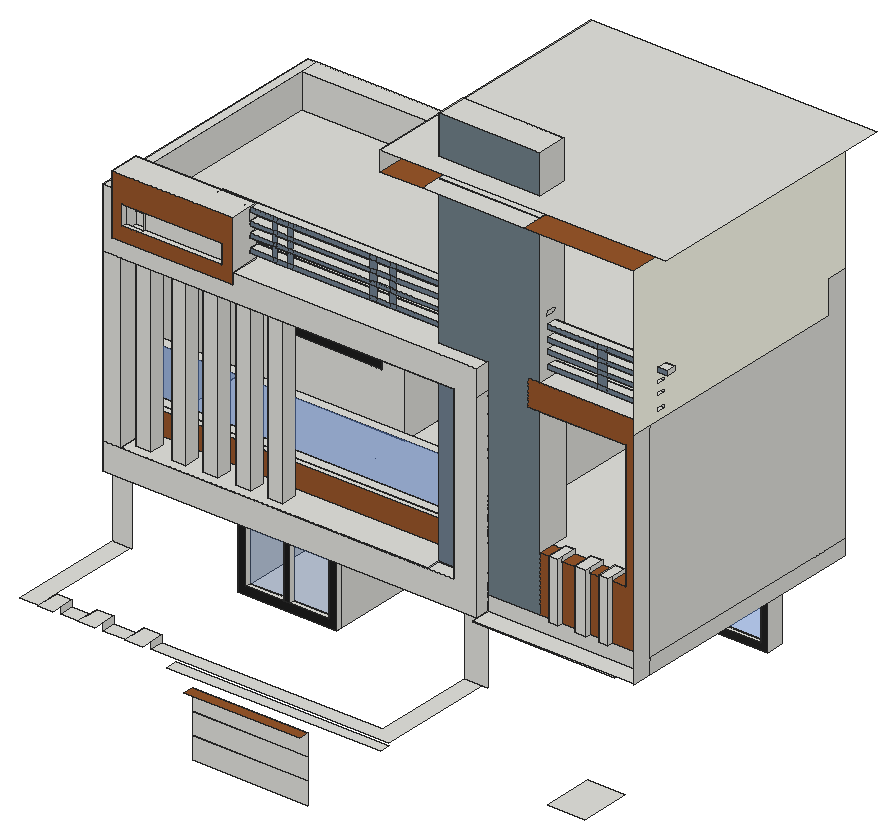
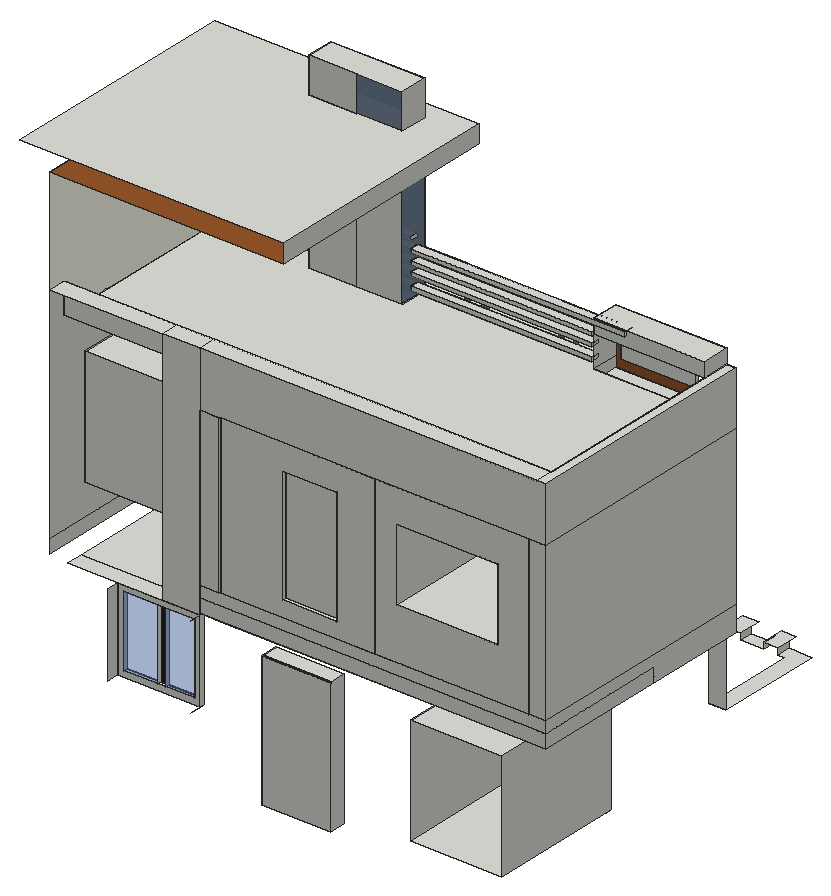
# SketchUp Ruby script. Lengths in inches.
U = 1.inch
M = Sketchup.active_model
def pt(a) = Geom::Point3d.new(a.map { |v| v * U })
def face(e, loops, mat)
  f = e.add_face(loops[0].map { |a| pt(a) })
  loops[1..].each { |l| e.add_face(l.map { |a| pt(a) }).erase! }
  f.material = f.back_material = mat if mat
  f
end
# faces: each face lists its corners as indices into pts; further lists are holes
def faces(e, pts, list, mat = nil) = list.each { |f| face(e, (f[0].is_a?(Array) ? f : [f]).map { |l| l.map { |i| pts[i] } }, mat) }
# xy, xz, yz: faces in a plane at the given z, y or x. An outline is a flat list of corners, or four numbers for a rectangle; further outlines are holes
def ring(l) = l.size == 4 ? [[l[0], l[1]], [l[2], l[1]], [l[2], l[3]], [l[0], l[3]]] : l.each_slice(2).to_a
def flat(e, list, mat, &to3) = list.each { |f| face(e, (f[0].is_a?(Array) ? f : [f]).map { |l| ring(l).map { |u, v| to3.(u, v) } }, mat) }
def xy(e, z, list, mat = nil) = flat(e, list, mat) { |x, y| [x, y, z] }
def xz(e, y, list, mat = nil) = flat(e, list, mat) { |x, z| [x, y, z] }
def yz(e, x, list, mat = nil) = flat(e, list, mat) { |y, z| [x, y, z] }
def lines(e, pts, list) = list.each { |a, b| e.add_line(pt(pts[a]), pt(pts[b])) }
# prism: a flat outline (further loops are holes) pulled along v
def prism(e, loops, v, mat = nil)
  f = face(e, loops, mat); d = Geom::Vector3d.new(v.map { |x| x * U })
  f.pushpull(f.normal.samedirection?(d) ? d.length : -d.length)
end
def box(e, o, s, mat = nil) = prism(e, [[o, [o[0] + s[0], o[1], o[2]], [o[0] + s[0], o[1] + s[1], o[2]], [o[0], o[1] + s[1], o[2]]]], [0, 0, s[2]], mat)
def at(x, y, z, deg = 0) = Geom::Transformation.translation(pt([x, y, z])) * Geom::Transformation.rotation(ORIGIN, Z_AXIS, deg.degrees)
def axes(o, x, y, z) = Geom::Transformation.new([*x, 0, *y, 0, *z, 0, *pt(o).to_a, 1])
def part(name) = M.definitions.add(name)
# library, detail: a bought-in or finely detailed component or shape, given as its bounding box
def library(name, o, s) = part(name).tap { |d| box(d.entities, o, s) }
def detail(e, o, s) = box(e.add_group.entities, o, s)
def put(e, d, t, mat = nil) = e.add_instance(d, t).tap { |i| i.material = mat if mat }
def group(e, t, mat = nil) = e.add_group.tap { |g| g.transformation = t; g.material = mat if mat }.entities
root = M.entities
M.materials.add("[0053_Ivory]").color = [255, 255, 240]
M.materials.add("[0111_SlateGray]").color = [112, 130, 152]
M.materials["[0111_SlateGray]"].alpha = 0.95
M.materials.add("[0111_SlateGray]1").color = [112, 128, 136]
M.materials.add("[0111_SlateGray]2").color = [112, 128, 144]
M.materials.add("[0136_Charcoal]").color = [35, 35, 35]
M.materials.add("[Color M08]").color = [30, 30, 30]
M.materials.add("[Translucent Glass Blue]").color = [100, 149, 237]
M.materials["[Translucent Glass Blue]"].alpha = 0.25
M.materials.add("[Translucent Glass Blue]1").color = [100, 149, 237]
M.materials["[Translucent Glass Blue]1"].alpha = 0.27
M.materials.add("[Translucent Glass Blue]2").color = [100, 149, 237]
M.materials["[Translucent Glass Blue]2"].alpha = 0.48
M.materials.add("[Translucent_Glass_Blue]1").color = [100, 149, 237]
M.materials["[Translucent_Glass_Blue]1"].alpha = 0.5
M.materials.add("[Wood Cherry Original]").color = [152, 86, 42]
c1 = part("DOOR12")
g1 = group(c1.entities,at(114.73,28.14,-0.51))
g2 = group(g1,at(0,0,0))
box(g2,[0,0,0],[36,0.5,77.7])
xy(root,4.04,[[120.48,208.05,157.11,217.05]])
xy(root,14.85,[[29.05,144.8,77.86,217.05]])
xy(root,40.28,[[90.86,34.4375,147.74,39.75]],"[Wood Cherry Original]")
xy(root,48.65,[[82.49,34.4375,187.77,39.75]])
xy(root,49.9375,[[5.71,39.75,18.06,39.75,18.06,46.62,14.21,46.62,14.21,97.05,5.71,97.05],[25.54,39.75,37.97,46.62],[46.56,39.75,61.07,46.62],[69.9,39.75,187.77,39.75,187.77,97.05,179.21,97.05,179.21,46.62,69.9,46.62],[265.92,39.75,284.23,64.5]])
xy(root,53.25,[[18.06,34.8125,25.54,46.62],[37.97,34.8125,46.56,46.62],[61.07,34.8125,69.9,46.62]])
xy(root,72.35,[[29.05,144.8,77.86,217.05]])
xy(root,75.48,[[120.48,208.05,157.11,217.05]])
xy(root,83.3,[[190.59,87.55,260.82,208.05],[190.59,208.05,260.82,217.05]])
xy(root,84,[[190.59,87.55,270.7,97.05],[5.71,97.05,14.71,144.8],[179.21,97.05,190.59,103.41],[179.21,103.41,190.59,144.8],[5.71,144.8,14.71,217.05],
  [14.71,144.8,96.96,217.05],[96.96,144.8,179.21,208.05],[179.21,144.8,190.59,208.05],[96.96,208.05,179.21,217.05],[179.21,208.05,190.59,217.05]])
xy(root,91.28,[[222.5,94.74,227.16,97.05],[235.14,94.74,240.98,97.05],[247.04,94.74,251.87,97.05],[5.71,144.8,190.59,217.05]])
xy(root,97.28,[[5.71,90.43,14.71,217.05],[14.71,90.43,14.71,144.8,96.96,144.8,96.96,208.05,179.21,208.05,179.21,97.05,166.45,97.05,166.45,90.43],[166.45,90.43,179.21,97.05],[180.15,97.05,190.59,217.05]])
xy(root,97.53,[[[14.71,90.43,166.45,90.43,166.45,97.05,179.21,97.05,179.21,208.05,96.96,208.05,96.96,163.18,14.71,163.18,14.71,110.21,168.09,110.21,168.09,107.46,14.71,107.46],[18.68,94.98,26.05,102.36],[36.05,94.98,43.43,102.36],[51.49,94.98,58.87,102.36],[67.93,94.98,75.3,102.36],[83.74,94.98,91.12,102.36]],[14.71,163.18,96.96,217.05],[96.96,208.05,179.21,217.05]])
xy(root,105.72,[[117.06,208.05,146.31,217.05]])
xy(root,109.03,[[14.71,107.46,168.09,110.21]])
xy(root,118.72,[[216.23,105.08,258.79,105.08,258.79,208.05,179.21,208.05,179.21,113.12,216.23,113.12]])
xy(root,118.72,[[216.23,97.05,222.5,105.08],[227.16,97.05,235.14,105.08],[240.98,97.05,247.04,105.08],[251.87,97.05,258.79,105.08]],"[Wood Cherry Original]")
xy(root,120.66,[[222.5,94.74,227.16,105.08],[235.14,94.74,240.98,105.08],[247.04,94.74,251.87,105.08]])
xy(root,124.87,[[31.09,163.18,85.47,217.05]])
xy(root,163.62,[[31.09,163.18,85.47,217.05]])
xy(root,167.65,[[117.06,208.05,146.31,217.05]])
xy(root,181.28,[[5.71,90.43,14.71,217.05],[[14.71,90.43,14.71,163.18,96.96,163.18,96.96,208.05,179.21,208.05,179.21,97.05,166.45,97.05,166.45,90.43],[83.74,94.98,91.12,102.36],[51.49,94.98,58.87,102.36],[18.68,94.98,26.05,102.36]],[166.45,90.43,179.21,97.05],[180.15,97.05,190.59,113.12],[210.17,97.05,216.23,113.12],
  [216.23,97.05,216.23,113.12,210.17,113.12,210.17,208.05,258.79,208.05,258.79,97.05],[179.21,113.12,180.15,208.05],[180.15,113.12,190.59,208.05],[190.59,113.12,210.17,208.05],[14.71,163.18,96.96,217.05],
  [96.96,208.05,179.21,217.05],[180.15,208.05,190.59,217.05]])
xy(root,183.03,[[36.05,94.98,43.43,102.36]])
xy(root,183.22,[[67.93,94.98,75.3,102.36]])
xy(root,188.5625,[[10.375,90.43,69.8125,105.06]])
xy(root,194.0625,[[69.8125,90.43,190.59,90.43,190.59,97.05,166.45,97.05,166.45,111.99,216.23,111.99,216.23,97.05,270.7,97.05,270.7,207.38,10.375,207.38,10.375,105.06,69.8125,105.06],[210.17,97.05,216.23,111.99]])
xy(root,195.77,[[15.47,90.43,24.35,92.37],[24.35,90.43,64.59,93.56]])
xy(root,198.07,[[69.8125,101.45,166.45,106.14],[166.45,101.45,216.23,106.14],[216.23,101.45,270.7,106.14]])
xy(root,200.2,[[69.8125,101.45,166.45,106.14],[166.45,101.45,216.23,106.14],[216.23,101.45,270.7,106.14]])
xy(root,204.88,[[69.8125,101.45,166.45,106.14],[166.45,101.45,216.23,106.14],[216.23,101.45,270.7,106.14]])
xy(root,205.27,[[15.47,90.43,24.35,92.37],[24.35,90.43,64.59,93.56]])
xy(root,207.01,[[69.8125,101.45,166.45,106.14],[166.45,101.45,216.23,106.14],[216.23,101.45,270.7,106.14]])
xy(root,210.2,[[69.8125,101.45,166.45,106.14],[166.45,101.45,216.23,106.14],[216.23,101.45,270.7,106.14]])
xy(root,210.6875,[[5.71,90.43,10.375,217.05],[10.375,207.38,190.59,217.05],[190.59,207.38,210.17,217.05],[210.17,207.38,270.7,217.05]])
xy(root,212.32,[[69.8125,101.45,166.45,106.14],[166.45,101.45,216.23,106.14],[216.23,101.45,270.7,106.14]])
xy(root,216.07,[[52.38,101.45,166.45,106.14],[166.45,101.45,216.23,106.14],[216.23,101.45,275.73,106.14]])
xy(root,218.2,[[52.38,101.45,166.45,106.14],[166.45,101.45,216.23,106.14],[216.23,101.45,275.73,106.14]])
xy(root,218.45,[[10.375,90.43,69.8125,105.06]])
xy(root,221.63,[[166.45,101.45,216.23,106.14]])
xy(root,223.76,[[166.45,101.45,216.23,106.14]])
xy(root,266.9,[[166.45,86.99,216.23,97.05],[166.45,97.05,216.23,111.99]])
xy(root,266.9,[[145.58,86.99,145.58,217.05,270.7,217.05,270.7,86.99,216.23,86.99,216.23,111.99,166.45,111.99,166.45,86.99]],"[Wood Cherry Original]")
xy(root,276.75,[[[145.58,86.99,286.33,217.05],[166.45,97.05,216.23,111.99]],[166.45,97.05,216.23,111.99]])
xy(root,295.6875,[[166.45,97.05,216.23,111.99]])
xz(root,39.75,[[90.86,8.21,147.74,18.9],[90.86,19.28,147.74,29.59],[90.86,29.9,147.74,40.28]])
xz(root,39.75,[[90.86,18.9,147.74,19.28],[90.86,29.59,147.74,29.9]],"[0136_Charcoal]")
xz(root,90.43,[[5.71,84,190.59,84,190.59,194.0625,69.8125,194.0625,69.8125,188.5625,10.375,188.5625,10.375,210.6875,5.71,210.6875,5.71,181.28,179.21,181.28,179.21,97.28,5.71,97.28],[5.71,97.28,14.71,181.28],[14.71,97.28,166.45,97.53]])
xz(root,90.43,[[[10.375,188.5625,69.8125,218.45],[15.47,195.77,64.59,205.27]]],"[Wood Cherry Original]")
xz(root,93.56,[[24.35,195.77,64.59,205.27]])
xz(root,94.74,[[222.5,91.28,227.16,120.66],[235.14,91.28,240.98,120.66],[247.04,91.28,251.87,120.66]])
xz(root,94.98,[[18.68,97.53,26.05,181.28],[36.05,97.53,43.43,183.03],[51.49,97.53,58.87,181.28],[67.93,97.53,75.3,183.22],[83.74,97.53,91.12,181.28]])
xz(root,97.05,[[5.71,49.9375,14.71,84],[179.21,49.9375,190.59,84],[190.59,84,270.7,91.28],[166.45,97.28,179.21,97.53],[180.15,97.28,190.59,181.28]])
xz(root,97.05,[[190.59,91.28,216.23,91.28,216.23,181.28,210.17,181.28,210.17,194.0625,216.23,194.0625,216.23,266.9,166.45,266.9,166.45,194.0625,190.59,194.0625],[166.45,276.75,216.23,295.6875]],"[0111_SlateGray]1")
xz(root,97.05,[[166.45,97.53,179.21,181.28]],"[0111_SlateGray]2")
xz(root,97.05,[[251.87,91.28,270.7,91.28,270.7,194.0625,210.17,194.0625,210.17,181.28,258.79,181.28,258.79,118.72,251.87,118.72],[216.23,91.28,222.5,118.72],[227.16,91.28,235.14,118.72],[240.98,91.28,247.04,118.72]],"[Wood Cherry Original]")
xz(root,101.45,[[166.45,198.07,216.23,200.2],[166.45,204.88,216.23,207.01],[166.45,210.2,216.23,212.32],[52.38,216.07,69.8125,218.2],[166.45,216.07,216.23,218.2],
  [166.45,221.63,216.23,223.76]])
xz(root,101.45,[[69.8125,198.07,80.96,200.2],[80.96,198.07,83.09,200.2],[83.09,198.07,88.54,200.2],[88.54,198.07,91.03,200.2],[91.03,198.07,128.74,200.2],
  [128.74,198.07,132.13,200.2],[132.13,198.07,138.62,200.2],[138.62,198.07,141.65,200.2],[141.65,198.07,166.45,200.2],[216.23,198.07,241.4,200.2],
  [241.4,198.07,245.98,200.2],[245.98,198.07,270.7,200.2],[80.96,200.2,83.09,204.88],[88.54,200.2,91.03,204.88],[128.74,200.2,132.13,204.88],
  [138.62,200.2,141.65,204.88],[241.4,200.2,245.98,204.88],[69.8125,204.88,80.96,207.01],[80.96,204.88,83.09,207.01],[83.09,204.88,88.54,207.01],
  [88.54,204.88,91.03,207.01],[91.03,204.88,128.74,207.01],[128.74,204.88,132.13,207.01],[132.13,204.88,138.62,207.01],[138.62,204.88,141.65,207.01],
  [141.65,204.88,166.45,207.01],[216.23,204.88,241.4,207.01],[241.4,204.88,245.98,207.01],[245.98,204.88,270.7,207.01],[80.96,207.01,83.09,210.2],
  [88.54,207.01,91.03,210.2],[128.74,207.01,132.13,210.2],[138.62,207.01,141.65,210.2],[241.4,207.01,245.98,210.2],[69.8125,210.2,80.96,212.32],
  [80.96,210.2,83.09,212.32],[83.09,210.2,88.54,212.32],[88.54,210.2,91.03,212.32],[91.03,210.2,128.74,212.32],[128.74,210.2,132.13,212.32],
  [132.13,210.2,138.62,212.32],[138.62,210.2,141.65,212.32],[141.65,210.2,166.45,212.32],[216.23,210.2,241.4,212.32],[241.4,210.2,245.98,212.32],
  [245.98,210.2,270.7,212.32],[80.96,212.32,83.09,216.07],[88.54,212.32,91.03,216.07],[128.74,212.32,132.13,216.07],[138.62,212.32,141.65,216.07],
  [241.4,212.32,245.98,216.07],[69.8125,216.07,80.96,218.2],[80.96,216.07,83.09,218.2],[83.09,216.07,88.54,218.2],[88.54,216.07,91.03,218.2],
  [91.03,216.07,128.74,218.2],[128.74,216.07,132.13,218.2],[132.13,216.07,138.62,218.2],[138.62,216.07,141.65,218.2],[141.65,216.07,166.45,218.2],
  [216.23,216.07,241.4,218.2],[241.4,216.07,245.98,218.2],[245.98,216.07,275.73,218.2]],"[0111_SlateGray]2")
xz(root,102.36,[[18.68,97.53,26.05,181.28],[36.05,97.53,43.43,183.03],[51.49,97.53,58.87,181.28],[67.93,97.53,75.3,183.22],[83.74,97.53,91.12,181.28]])
xz(root,105.06,[[10.375,188.5625,69.8125,194.0625],[10.375,210.6875,69.8125,218.45]])
xz(root,105.08,[[222.5,118.72,227.16,120.66],[235.14,118.72,240.98,120.66],[247.04,118.72,251.87,120.66]])
xz(root,106.14,[[69.8125,198.07,166.45,200.2],[166.45,198.07,216.23,200.2],[216.23,198.07,270.7,200.2],[69.8125,204.88,166.45,207.01],[166.45,204.88,216.23,207.01],
  [216.23,204.88,270.7,207.01],[69.8125,210.2,166.45,212.32],[166.45,210.2,216.23,212.32],[216.23,210.2,270.7,212.32],[52.38,216.07,166.45,218.2],
  [166.45,216.07,216.23,218.2],[216.23,216.07,275.73,218.2],[166.45,221.63,216.23,223.76]])
xz(root,107.46,[[14.71,97.53,168.09,109.03]],"[Wood Cherry Original]")
xz(root,110.21,[[14.71,97.53,168.09,109.03]])
xz(root,111.99,[[166.45,194.0625,190.59,266.9],[190.59,194.0625,216.23,266.9],[190.59,266.9,216.23,276.75],[190.59,276.75,216.23,295.6875]])
xz(root,111.99,[[166.45,266.9,190.59,276.75],[166.45,276.75,190.59,295.6875]],"[0111_SlateGray]")
xz(root,113.12,[[179.21,118.72,216.23,181.28]])
xz(root,144.8,[[5.71,84,190.59,91.28]])
xz(root,163.18,[[[14.71,97.53,96.96,181.28],[31.09,124.87,85.47,163.62]]])
xz(root,207.38,[[10.375,194.0625,270.7,210.6875]])
xz(root,208.05,[[96.96,97.28,179.21,97.53],[[96.96,97.53,179.21,181.28],[117.06,105.72,146.31,167.65]],[117.06,105.72,146.31,167.65],[179.21,118.72,258.79,181.28]])
xz(root,217.05,[[190.59,83.3,210.17,210.6875],[5.71,84,190.59,91.28],[5.71,91.28,190.59,97.28],[5.71,97.28,14.71,181.28],[180.15,97.28,190.59,181.28],
  [[14.71,97.53,96.96,181.28],[31.09,124.87,85.47,163.62]],[[96.96,97.53,179.21,181.28],[117.06,105.72,146.31,167.65]],[5.71,181.28,190.59,210.6875]])
yz(root,5.71,[[90.43,84,90.43,97.28,217.05,97.28,217.05,91.28,144.8,91.28,144.8,84],[144.8,84,217.05,91.28],[90.43,97.28,217.05,181.28],[90.43,181.28,217.05,210.6875]])
yz(root,10.375,[[90.43,188.5625,105.06,210.6875],[105.06,194.0625,207.38,210.6875],[90.43,210.6875,105.06,218.45]])
yz(root,14.71,[[90.43,97.28,107.46,97.53],[107.46,97.28,117.62,97.28,117.62,97.53,110.21,97.53,110.21,109.03,107.46,109.03],[144.8,97.28,217.05,97.53],[90.43,97.53,107.46,97.53,107.46,109.03,110.21,109.03,110.21,97.53,163.18,97.53,163.18,181.28,90.43,181.28],[163.18,97.53,217.05,181.28]])
yz(root,15.47,[[90.43,195.77,92.37,205.27]])
yz(root,18.06,[[39.75,49.9375,46.62,53.25]])
yz(root,18.68,[[94.98,97.53,102.36,181.28]])
yz(root,24.35,[[92.37,195.77,93.56,205.27]])
yz(root,25.54,[[39.75,49.9375,46.62,53.25]])
yz(root,26.05,[[94.98,97.53,102.36,181.28]])
yz(root,29.05,[[144.8,14.85,217.05,72.35]])
yz(root,31.09,[[163.18,124.87,217.05,163.62]])
yz(root,36.05,[[94.98,97.53,102.36,183.03]])
yz(root,37.97,[[39.75,49.9375,46.62,53.25]])
yz(root,43.43,[[94.98,97.53,102.36,183.03]])
yz(root,46.56,[[39.75,49.9375,46.62,53.25]])
yz(root,51.49,[[94.98,97.53,102.36,181.28]])
yz(root,52.38,[[101.45,216.07,106.14,218.2]])
yz(root,58.87,[[94.98,97.53,102.36,181.28]])
yz(root,61.07,[[39.75,49.9375,46.62,53.25]])
yz(root,64.59,[[90.43,195.77,93.56,205.27]])
yz(root,67.93,[[94.98,97.53,102.36,183.22]])
yz(root,69.8125,[[90.43,188.5625,105.06,194.0625],[90.43,194.0625,105.06,194.0625,105.06,198.07,101.45,198.07,101.45,200.2,105.06,200.2,105.06,204.88,101.45,204.88,101.45,207.01,105.06,207.01,105.06,210.2,101.45,210.2,101.45,218.45,90.43,218.45],[101.45,198.07,105.06,200.2],[105.06,198.07,106.14,200.2],[101.45,204.88,105.06,207.01],
  [105.06,204.88,106.14,207.01],[101.45,210.2,105.06,212.32],[105.06,210.2,106.14,212.32],[101.45,212.32,105.06,218.45]])
yz(root,69.9,[[39.75,49.9375,46.62,53.25]])
yz(root,75.3,[[94.98,97.53,102.36,183.22]])
yz(root,77.86,[[144.8,14.85,217.05,72.35]])
yz(root,83.74,[[94.98,97.53,102.36,181.28]])
yz(root,85.47,[[163.18,124.87,217.05,163.62]])
yz(root,91.12,[[94.98,97.53,102.36,181.28]])
yz(root,96.96,[[163.18,97.53,208.05,181.28],[208.05,97.53,217.05,181.28]])
yz(root,117.06,[[208.05,105.72,217.05,167.65]])
yz(root,120.48,[[208.05,4.04,217.05,75.48]])
yz(root,145.58,[[86.99,266.9,217.05,276.75]])
yz(root,146.31,[[208.05,105.72,217.05,167.65]])
yz(root,157.11,[[208.05,4.04,217.05,75.48]])
yz(root,166.45,[[90.43,97.28,97.05,97.53],[97.05,188.5625,111.99,194.0625],[101.45,198.07,106.14,200.2],[101.45,204.88,106.14,207.01],[101.45,210.2,106.14,212.32],
  [101.45,216.07,106.14,218.2],[101.45,221.63,106.14,223.76],[97.05,276.75,111.99,295.6875]])
yz(root,166.45,[[[97.05,194.0625,111.99,266.9],[101.45,221.63,106.14,223.76],[101.45,216.07,106.14,218.2],[101.45,210.2,106.14,212.32],[101.45,204.88,106.14,207.01],[101.45,198.07,106.14,200.2]]],"[0111_SlateGray]")
yz(root,168.09,[[107.46,97.53,110.21,109.03]])
yz(root,179.21,[[90.43,97.28,97.05,181.28],[97.05,97.28,208.05,97.53],[97.05,97.53,97.05,181.28,113.12,181.28,113.12,118.72,208.05,118.72,208.05,97.53],[208.05,97.53,217.05,112.03],[208.05,112.03,217.05,181.28]])
yz(root,180.15,[[97.05,97.28,217.05,181.28]])
yz(root,190.59,[[87.55,83.3,97.05,84],[103.41,83.3,208.05,84],[208.05,83.3,217.05,84],[90.43,84,97.05,181.28],[97.05,84,144.8,84,144.8,91.28,217.05,91.28,217.05,97.28,97.05,97.28],
  [144.8,84,217.05,91.28],[97.05,97.28,217.05,181.28],[90.43,181.28,97.05,194.0625]])
yz(root,216.23,[[97.05,118.72,113.12,181.28],[[97.05,194.0625,111.99,266.9],[101.45,221.63,106.14,223.76],[101.45,216.07,106.14,218.2],[101.45,210.2,106.14,212.32],[101.45,204.88,106.14,207.01],[101.45,198.07,106.14,200.2]],[101.45,221.63,106.14,223.76],[97.05,276.75,111.99,295.6875]])
yz(root,222.5,[[94.74,91.28,97.05,120.66],[97.05,118.72,105.08,120.66]])
yz(root,227.16,[[94.74,91.28,97.05,120.66],[97.05,118.72,105.08,120.66]])
yz(root,235.14,[[94.74,91.28,97.05,120.66],[97.05,118.72,105.08,120.66]])
yz(root,239.77,[[208.05,34.28,217.05,78.41]])
yz(root,240.98,[[94.74,91.28,97.05,120.66],[97.05,118.72,105.08,120.66]])
yz(root,247.04,[[94.74,91.28,97.05,120.66],[97.05,118.72,105.08,120.66]])
yz(root,251.87,[[94.74,91.28,97.05,120.66],[97.05,118.72,105.08,120.66]])
yz(root,258.79,[[97.05,118.72,208.05,181.28]])
yz(root,270.7,[[86.99,84,97.05,194.0625],[97.05,84,217.05,91.28],[97.05,91.28,217.05,91.28,217.05,210.6875,207.38,210.6875,207.38,194.0625,97.05,194.0625]])
yz(root,270.7,[[[86.99,194.0625,86.99,266.9,217.05,266.9,217.05,210.6875,207.38,210.6875,207.38,194.0625],[101.45,210.2,106.14,212.32],[101.45,204.88,106.14,207.01],[101.45,198.07,106.14,200.2]]],"[0053_Ivory]")
yz(root,275.73,[[101.45,216.07,106.14,218.2]])
p = [[210.17,208.05,105.53],[210.17,217.05,105.53],[210.17,208.05,181.28],[210.17,217.05,181.28],[96.96,144.8,97.53],[96.96,144.8,97.28],
  [195.64,208.05,78.41],[195.64,217.05,78.41],[195.64,208.05,34.28],[195.64,217.05,34.28]]
lines(root,p,[[0,1],[2,3],[4,5],[6,7],[8,9]])
put(root,c1,axes([3.76,180.31,4.51],[1.01736,0,0],[0,1.2831,0],[0,0,0.91943]))
g3 = group(root,at(29.05,144.8,14.85))
xy(g3,0,[[0,0,48.8125,2.625]])
xy(g3,3.92,[[3.92,0,22.65,2.625],[22.65,0,25.47,2.625],[25.47,0,44.89,2.625]])
xy(g3,53.58,[[3.92,0,22.65,2.625],[22.65,0,25.47,2.625],[25.47,0,44.89,2.625]])
xy(g3,57.5,[[0,0,48.8125,2.625]])
xz(g3,0,[[[0,0,48.8125,57.5],[3.92,3.92,44.89,53.58]],[22.65,3.92,25.47,53.58]],"[Color M08]")
xz(g3,2.625,[[[0,0,48.8125,57.5],[3.92,3.92,44.89,53.58]]])
xz(g3,2.625,[[3.92,3.92,22.65,53.58],[25.47,3.92,44.89,53.58]],"[Translucent Glass Blue]1")
yz(g3,0,[[0,0,2.625,57.5]])
yz(g3,3.92,[[0,3.92,2.625,53.58]])
yz(g3,22.65,[[0,3.92,2.625,53.58]])
yz(g3,25.47,[[0,3.92,2.625,53.58]])
yz(g3,44.89,[[0,3.92,2.625,53.58]])
yz(g3,48.8125,[[0,0,2.625,57.5]])
g4 = group(root,at(195.64,208.05,34.28))
xy(g4,0,[[0,0,44.125,2.1875]])
xy(g4,3.11,[[3.11,0,18.59,2.1875],[18.59,0,22.72,2.1875],[22.72,0,41.02,2.1875]])
xy(g4,41.02,[[3.11,0,18.59,2.1875],[18.59,0,22.72,2.1875],[22.72,0,41.02,2.1875]])
xy(g4,44.125,[[0,0,44.125,2.1875]])
xz(g4,0,[[[0,0,44.125,44.125],[3.11,3.11,41.02,41.02]],[18.59,3.11,22.72,41.02]],"[0136_Charcoal]")
xz(g4,2.1875,[[[0,0,44.125,44.125],[3.11,3.11,41.02,41.02]]])
xz(g4,2.1875,[[3.11,3.11,18.59,41.02],[22.72,3.11,41.02,41.02]],"[Translucent Glass Blue]2")
yz(g4,0,[[0,0,2.1875,44.125]])
yz(g4,3.11,[[0,3.11,2.1875,41.02]])
yz(g4,18.59,[[0,3.11,2.1875,41.02]])
yz(g4,22.72,[[0,3.11,2.1875,41.02]])
yz(g4,41.02,[[0,3.11,2.1875,41.02]])
yz(g4,44.125,[[0,0,2.1875,44.125]])
put(root,c1,axes([23.84,-161.33,106.125],[0.8125,0,0],[0,13.1274,0],[0,0,0.79716]))
g5 = group(root,at(14.71,114.86,109.03))
xy(g5,0,[[0,-4.42,151.73,0]])
xy(g5,26.46,[[0,-4.42,151.73,0]])
xz(g5,0,[[0,0,151.73,26.46]],"[Translucent_Glass_Blue]1")
yz(g5,0,[[-4.42,0,0,26.46]])
yz(g5,151.73,[[-4.42,0,0,26.46]])
g6 = group(root,at(31.09,163.18,124.87))
xz(g6,0,[[[0,0,54.375,38.75],[4.65,4.65,49.72,34.1]],[27.1875,4.65,29.5,34.1]],"[Color M08]")
xz(g6,0,[[4.65,4.65,27.1875,34.1],[29.5,4.65,49.72,34.1]],"[Translucent Glass Blue]")
